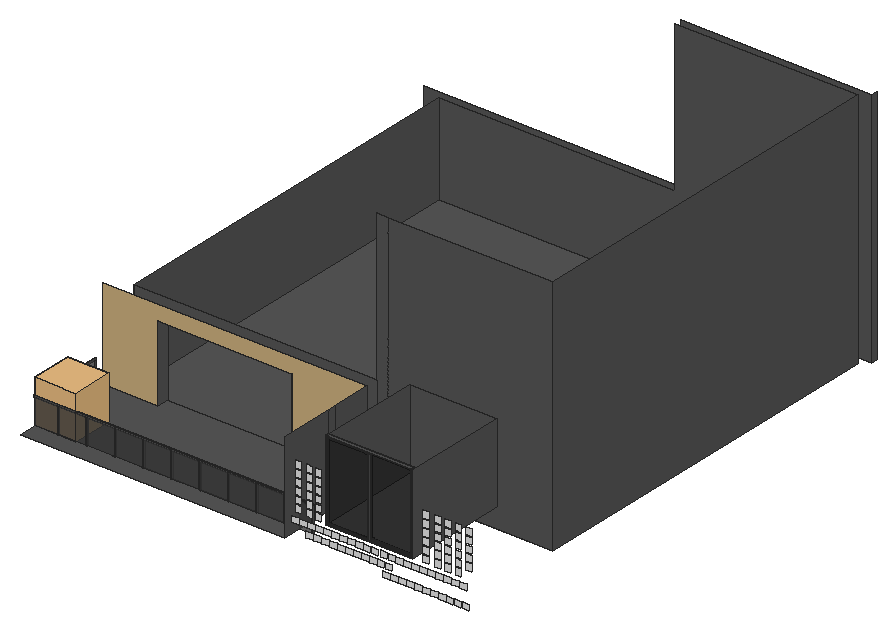
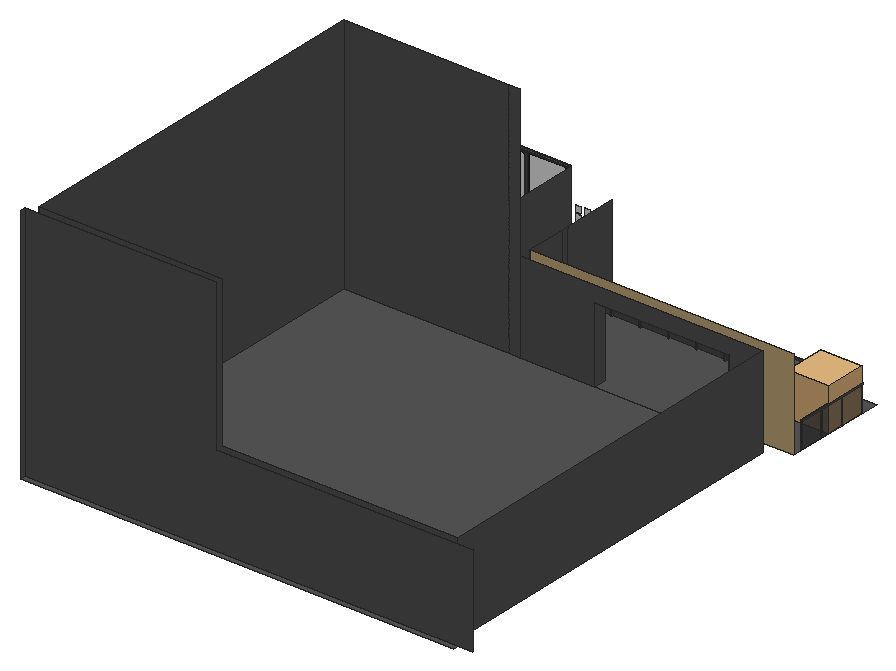
# SketchUp Ruby script. Lengths in inches.
U = 1.inch
M = Sketchup.active_model
def pt(a) = Geom::Point3d.new(a.map { |v| v * U })
def face(e, loops, mat)
  f = e.add_face(loops[0].map { |a| pt(a) })
  loops[1..].each { |l| e.add_face(l.map { |a| pt(a) }).erase! }
  f.material = f.back_material = mat if mat
  f
end
# faces: each face lists its corners as indices into pts; further lists are holes
def faces(e, pts, list, mat = nil) = list.each { |f| face(e, (f[0].is_a?(Array) ? f : [f]).map { |l| l.map { |i| pts[i] } }, mat) }
# xy, xz, yz: faces in a plane at the given z, y or x. An outline is a flat list of corners, or four numbers for a rectangle; further outlines are holes
def ring(l) = l.size == 4 ? [[l[0], l[1]], [l[2], l[1]], [l[2], l[3]], [l[0], l[3]]] : l.each_slice(2).to_a
def flat(e, list, mat, &to3) = list.each { |f| face(e, (f[0].is_a?(Array) ? f : [f]).map { |l| ring(l).map { |u, v| to3.(u, v) } }, mat) }
def xy(e, z, list, mat = nil) = flat(e, list, mat) { |x, y| [x, y, z] }
def xz(e, y, list, mat = nil) = flat(e, list, mat) { |x, z| [x, y, z] }
def yz(e, x, list, mat = nil) = flat(e, list, mat) { |y, z| [x, y, z] }
def lines(e, pts, list) = list.each { |a, b| e.add_line(pt(pts[a]), pt(pts[b])) }
# prism: a flat outline (further loops are holes) pulled along v
def prism(e, loops, v, mat = nil)
  f = face(e, loops, mat); d = Geom::Vector3d.new(v.map { |x| x * U })
  f.pushpull(f.normal.samedirection?(d) ? d.length : -d.length)
end
def box(e, o, s, mat = nil) = prism(e, [[o, [o[0] + s[0], o[1], o[2]], [o[0] + s[0], o[1] + s[1], o[2]], [o[0], o[1] + s[1], o[2]]]], [0, 0, s[2]], mat)
def at(x, y, z, deg = 0) = Geom::Transformation.translation(pt([x, y, z])) * Geom::Transformation.rotation(ORIGIN, Z_AXIS, deg.degrees)
def axes(o, x, y, z) = Geom::Transformation.new([*x, 0, *y, 0, *z, 0, *pt(o).to_a, 1])
def part(name) = M.definitions.add(name)
# library, detail: a bought-in or finely detailed component or shape, given as its bounding box
def library(name, o, s) = part(name).tap { |d| box(d.entities, o, s) }
def detail(e, o, s) = box(e.add_group.entities, o, s)
def put(e, d, t, mat = nil) = e.add_instance(d, t).tap { |i| i.material = mat if mat }
def group(e, t, mat = nil) = e.add_group.tap { |g| g.transformation = t; g.material = mat if mat }.entities
root = M.entities
M.materials.add("Glass_Tinted_Gray").color = [0, 0, 0]
M.materials["Glass_Tinted_Gray"].alpha = 0.125
M.materials.add("[0135_DarkGray]").color = [81, 81, 81]
M.materials.add("[Color M06]").color = [86, 86, 86]
M.materials.add("[Mirror 02]").color = [229, 229, 229]
M.materials.add("[Polished Concrete Old]").color = [229, 229, 229]
M.materials.add("[Terrazzo Light Blue]").color = [196, 214, 227]
M.materials.add("[Translucent Glass Safety]").color = [204, 235, 244]
M.materials["[Translucent Glass Safety]"].alpha = 0.5
M.materials.add("[Translucent_Glass_Gray]").color = [63, 63, 63]
M.materials["[Translucent_Glass_Gray]"].alpha = 0.54
M.materials.add("[Wood Floor Light]").color = [204, 176, 127]
c1 = library("Pot+Plant",[-20.81,-17.08,-0.03],[39.86,39.43,41.33])
c2 = part("Group\#81")
box(c2.entities,[0,0,0],[0.79,39.37,35.43],"[Translucent_Glass_Gray]")
c3 = part("Group\#82")
box(c3.entities,[0,0,0],[0.59,1.57,34.25])
c4 = part("Group\#85")
g1 = group(c4.entities,at(0.55,0.5,0))
put(g1,c2,axes([293.06,0,0],[0,0.84,0],[-0.92977,0,0],[0,0,1]),"[Translucent Glass Safety]")
g2 = group(g1,at(0,33.57,0),"[Translucent Glass Safety]")
box(g2,[0,0,0],[0.73,33.07,35.43],"[Translucent_Glass_Gray]")
put(g1,c2,axes([218.38,0,0],[0,0.84,0],[-0.92977,0,0],[0,0,1]),"[Translucent Glass Safety]")
put(g1,c2,axes([367.73,0,0],[0,0.84,0],[-0.92977,0,0],[0,0,1]),"[Translucent Glass Safety]")
g3 = group(g1,at(31.69,0,0),"[Translucent Glass Safety]")
box(g3,[-30.96,0,0],[30.96,0.66,35.43],"[Translucent_Glass_Gray]")
put(g1,c2,axes([255.72,0,0],[0,0.84,0],[-0.92977,0,0],[0,0,1]),"[Translucent Glass Safety]")
g4 = group(g1,at(181.04,0,0),"[Translucent Glass Safety]")
box(g4,[-36.61,0,0],[36.61,0.66,35.43],"[Translucent_Glass_Gray]")
g5 = group(g1,at(0,0.66,0),"[Translucent Glass Safety]")
box(g5,[0,0,0],[0.73,32.24,35.43],"[Translucent_Glass_Gray]")
g6 = group(g1,at(143.71,0,0),"[Translucent Glass Safety]")
box(g6,[-36.61,0,0],[36.61,0.66,35.43],"[Translucent_Glass_Gray]")
g7 = group(g1,at(69.03,0,0),"[Translucent Glass Safety]")
box(g7,[-36.61,0,0],[36.61,0.66,35.43],"[Translucent_Glass_Gray]")
g8 = group(g1,at(0,67.3,0),"[Translucent Glass Safety]")
box(g8,[0,0,0],[0.73,33.07,35.43],"[Translucent_Glass_Gray]")
put(g1,c3,axes([107.44,0.66,0],[0,1,0],[-0.92977,0,0],[0,0,1]),"[0135_DarkGray]")
put(g1,c3,axes([144.78,0.66,0],[0,1,0],[-0.92977,0,0],[0,0,1]),"[0135_DarkGray]")
put(g1,c3,axes([182.11,0.66,0],[0,1,0],[-0.92977,0,0],[0,0,1]),"[0135_DarkGray]")
put(g1,c3,axes([256.79,0.66,0],[0,1,0],[-0.92977,0,0],[0,0,1]),"[0135_DarkGray]")
put(g1,c3,axes([368.14,0.66,0],[0,1,0],[-0.92977,0,0],[0,0,1]),"[0135_DarkGray]")
put(g1,c3,axes([0.73,98.83,0],[0.92977,0,0],[0,1,0],[0,0,1]),"[0135_DarkGray]")
put(g1,c3,axes([331.46,0.66,0],[0,1,0],[-0.92977,0,0],[0,0,1]),"[0135_DarkGray]")
g9 = group(g1,at(106.37,0,0),"[Translucent Glass Safety]")
box(g9,[-36.61,0,0],[36.61,0.66,35.43],"[Translucent_Glass_Gray]")
put(g1,c2,axes([330.39,0,0],[0,0.84,0],[-0.92977,0,0],[0,0,1]),"[Translucent Glass Safety]")
put(g1,c3,axes([294.125,0.66,0],[0,1,0],[-0.92977,0,0],[0,0,1]),"[0135_DarkGray]")
put(g1,c3,axes([0.73,66.04,0],[0.92977,0,0],[0,1,0],[0,0,1]),"[0135_DarkGray]")
put(g1,c3,axes([0.73,32.31,0],[0.92977,0,0],[0,1,0],[0,0,1]),"[0135_DarkGray]")
put(g1,c3,axes([32.76,0.66,0],[0,1,0],[-0.92977,0,0],[0,0,1]),"[0135_DarkGray]")
put(g1,c3,axes([70.1,0.66,0],[0,1,0],[-0.92977,0,0],[0,0,1]),"[0135_DarkGray]")
put(g1,c3,axes([219.45,0.66,0],[0,1,0],[-0.92977,0,0],[0,0,1]),"[0135_DarkGray]")
g10 = group(c4.entities,at(0,0,34.25))
xy(g10,0,[[0,0,0,100.87,0.55,100.87,0.55,0.5,362.73,0.5,362.73,0],[362.73,0,369.35,0.5],[368.19,0.5,368.6875,1.16],[1.28,1.16,1.28,100.87,1.83,100.87,1.83,1.65,362.73,1.65,362.73,1.16],[362.73,1.16,368.19,1.65]],"[0135_DarkGray]")
xy(g10,1.18,[[368.19,0,368.6875,0.5],[368.6875,0,369.35,0.5],[0.55,0.5,0.55,100.87,1.28,100.87,1.28,1.16,362.73,1.16,362.73,0.5],[368.6875,0.5,369.35,1.16]],"[0135_DarkGray]")
xy(g10,1.97,[[0,0,362.73,0,362.73,1.65,1.83,1.65,1.83,100.87,0,100.87],[362.73,0,368.19,1.65]],"[0135_DarkGray]")
xz(g10,0,[[0,0,362.73,1.97],[362.73,0,369.35,0,369.35,1.18,368.19,1.18,368.19,1.97,362.73,1.97]],"[0135_DarkGray]")
xz(g10,0.5,[[0.55,0,1.28,1.18],[1.28,0,362.73,1.18],[362.73,0,368.19,1.18],[368.19,0,368.6875,1.18],[368.6875,0,369.35,1.18]],"[0135_DarkGray]")
xz(g10,1.16,[[1.28,0,362.73,1.18],[362.73,0,368.19,1.18]],"[0135_DarkGray]")
xz(g10,1.65,[[1.83,0,362.73,1.97],[362.73,0,368.19,1.97]],"[0135_DarkGray]")
xz(g10,100.87,[[0,0,0,1.97,1.83,1.97,1.83,0,1.28,0,1.28,1.18,0.55,1.18,0.55,0]],"[0135_DarkGray]")
yz(g10,0,[[0,0,100.87,1.97]],"[0135_DarkGray]")
yz(g10,0.55,[[0.5,0,100.87,1.18]],"[0135_DarkGray]")
yz(g10,1.28,[[1.16,0,100.87,1.18]],"[0135_DarkGray]")
yz(g10,1.83,[[1.65,0,100.87,1.97]],"[0135_DarkGray]")
yz(g10,362.73,[[0,0,0,1.97,1.65,1.97,1.65,0,1.16,0,1.16,1.18,0.5,1.18,0.5,0]],"[0135_DarkGray]")
yz(g10,368.19,[[1.16,0,1.65,0,1.65,1.97,0,1.97,0,1.18,1.16,1.18],[0.5,0,1.16,1.18]],"[0135_DarkGray]")
yz(g10,368.6875,[[0.5,0,1.16,1.18]],"[0135_DarkGray]")
yz(g10,369.35,[[0,0,0.5,1.18]],"[0135_DarkGray]")
c5 = part("PENTEK_RP Fineline 50S_Sliding_DoorCase_E1")
box(c5.entities,[0,0,0],[1.51,3.66,99.27],"[0135_DarkGray]")
c6 = part("PENTEK_RP Fineline 50S_SlidingDooe_Case_E2")
box(c6.entities,[0,0,0],[96.25,3.66,1.51],"[0135_DarkGray]")
c7 = part("pentek_RP Fineline 50S_SlidingDoor_Case")
put(c7.entities,c5,at(97.76,0,0))
put(c7.entities,c6,at(1.51,0,0))
put(c7.entities,c5,at(0,0,0))
put(c7.entities,c6,at(1.51,0,97.76))
c8 = part("PENTEK_RP Fineline 50S_SlidingDoor_GlazingBead_2")
box(c8.entities,[0,0,0],[0.56,0.59,94.39],"[0135_DarkGray]")
c9 = part("PENTEK_RP Fineline 50S_SlidingDoor_Glass")
box(c9.entities,[0,0,0],[46.58,0.16,94.39],"Glass_Tinted_Gray")
c10 = part("PENTEK_RP Fineline 50S_SlidingDoor_GlazingBead")
box(c10.entities,[0,0,0],[45.47,0.59,0.56],"[0135_DarkGray]")
c11 = part("PENTEK_RP Fineline 50S_SlidingDoor_Leaf_E1")
xy(c11.entities,0,[[0,0,0.93,1.97],[0.93,1.57,1.49,1.97]],"[0135_DarkGray]")
xy(c11.entities,96.25,[[0,0,0.93,0,0.93,1.57,1.49,1.57,1.49,1.97,0,1.97]],"[0135_DarkGray]")
xz(c11.entities,0,[[0,0,0.93,96.25]],"[0135_DarkGray]")
xz(c11.entities,1.57,[[0.93,0,1.49,95.32],[0.93,95.32,1.49,96.25]],"[0135_DarkGray]")
xz(c11.entities,1.97,[[0,0,1.49,96.25]],"[0135_DarkGray]")
yz(c11.entities,0,[[0,0,1.97,96.25]],"[0135_DarkGray]")
yz(c11.entities,0.93,[[0,0,1.57,0.93],[0,0.93,1.57,95.32],[0,95.32,1.57,96.25]],"[0135_DarkGray]")
yz(c11.entities,1.49,[[1.57,0,1.97,95.32],[1.57,95.32,1.97,96.25]],"[0135_DarkGray]")
c12 = part("PENTEK_RP Fineline 50S_SlidingDoor_Leaf_E2")
xy(c12.entities,0,[[0,0,0,1.57,0.56,1.57,0.56,1.97,46.02,1.97,46.02,1.57,46.58,1.57,46.58,0]],"[0135_DarkGray]")
xy(c12.entities,0.93,[[0,0,46.58,1.57]],"[0135_DarkGray]")
xy(c12.entities,1.49,[[0.56,1.57,46.02,1.97]],"[0135_DarkGray]")
xz(c12.entities,0,[[0,0,46.58,0.93]],"[0135_DarkGray]")
xz(c12.entities,1.57,[[0,0,0.56,0.93],[46.02,0,46.58,0.93],[0.56,0.93,46.02,1.49]],"[0135_DarkGray]")
xz(c12.entities,1.97,[[0.56,0,46.02,1.49]],"[0135_DarkGray]")
yz(c12.entities,0,[[0,0,1.57,0.93]],"[0135_DarkGray]")
yz(c12.entities,0.56,[[1.57,0,1.97,0.93],[1.57,0.93,1.97,1.49]],"[0135_DarkGray]")
yz(c12.entities,46.02,[[1.57,0,1.97,0.93],[1.57,0.93,1.97,1.49]],"[0135_DarkGray]")
yz(c12.entities,46.58,[[0,0,1.57,0.93]],"[0135_DarkGray]")
c13 = part("PENTEK_RP Fineline S_SlidingDoor_Leaf1")
put(c13.entities,c8,at(0.93,0,0.93))
put(c13.entities,c8,at(46.96,0,0.93))
put(c13.entities,c9,at(1.49,1.42,0.93))
put(c13.entities,c10,at(1.49,0,0.93))
put(c13.entities,c9,at(1.49,0.59,0.93),"[Terrazzo Light Blue]")
put(c13.entities,c11,at(0,0,0))
put(c13.entities,c11,axes([48.44,0,0],[-1,0,0],[0,1,0],[0,0,1]))
put(c13.entities,c12,axes([0.93,0,96.25],[1,0,0],[0,1,0],[0,0,-1]))
put(c13.entities,c12,at(0.93,0,0))
put(c13.entities,c10,at(1.49,0,94.77))
c14 = part("PENTEK_RP Fineline 50S_SlidingDoor_Leaf2")
put(c14.entities,c9,at(1.49,1.42,0.93))
put(c14.entities,c10,at(1.49,0,94.77))
put(c14.entities,c8,at(46.96,0,0.93))
put(c14.entities,c9,at(1.49,0.59,0.93),"[Mirror 02]")
put(c14.entities,c8,at(0.93,0,0.93))
put(c14.entities,c11,at(0,0,0))
put(c14.entities,c11,axes([48.44,0,0],[-1,0,0],[0,1,0],[0,0,1]))
put(c14.entities,c10,at(1.49,0,0.93))
put(c14.entities,c12,axes([0.93,0,96.25],[1,0,0],[0,1,0],[0,0,-1]))
put(c14.entities,c12,at(0.93,0,0))
c15 = part("PENTEK - Slimmest Steel Sliding Door / Window\#1")
put(c15.entities,c7,at(0,-1.88,-0.09))
put(c15.entities,c13,at(1.51,-2.27,1.42))
put(c15.entities,c14,at(49.32,-0.3,1.42))
xy(root,257.83,[[1.28,10.05,349.9,10.05,349.9,145.99,250.86,145.99,250.86,161.89,74.05,161.89,74.05,145.99,1.28,145.99],[29.53,161.89,582.75,665.33],[19.84,675.01,592.4375,683.05]],"[Color M06]")
xy(root,292.65,[[404.15,10.05,518.59,148.99]],"[Color M06]")
xz(root,10.05,[[479.61,257.42,488.61,264.73],[490.11,257.42,499.11,264.73],[500.61,257.42,509.61,264.73],[511.11,257.42,520.11,264.73],[521.61,257.42,530.61,264.73],
  [532.11,257.42,541.11,264.73],[542.61,257.42,551.61,264.73],[553.11,257.42,562.11,264.73],[563.61,257.42,572.61,264.73],[574.11,257.42,583.11,264.73],
  [584.61,257.42,593.61,264.73],[378.09,268.5,387.09,275.81],[388.59,268.5,397.59,275.81],[399.09,268.5,408.09,275.81],[409.59,268.5,418.59,275.81],
  [420.09,268.5,429.09,275.81],[430.59,268.5,439.59,275.81],[441.09,268.5,450.09,275.81],[451.59,268.5,460.59,275.81],[462.09,268.5,471.09,275.81],
  [472.59,268.5,481.59,275.81],[483.09,268.5,492.09,275.81],[359.62,280.4375,368.62,287.75],[370.12,280.4375,379.12,287.75],[380.62,280.4375,389.62,287.75],
  [391.12,280.4375,400.12,287.75],[401.62,280.4375,410.62,287.75],[412.12,280.4375,421.12,287.75],[422.62,280.4375,431.62,287.75],[433.12,280.4375,442.12,287.75],
  [443.62,280.4375,452.62,287.75],[454.12,280.4375,463.12,287.75],[464.62,280.4375,473.62,287.75],[476.43,280.4375,485.43,287.75],[486.93,280.4375,495.93,287.75],
  [497.43,280.4375,506.43,287.75],[507.93,280.4375,516.93,287.75],[518.43,280.4375,527.43,287.75],[528.93,280.4375,537.93,287.75],[539.43,280.4375,548.43,287.75],
  [549.93,280.4375,558.93,287.75],[560.43,280.4375,569.43,287.75],[570.93,280.4375,579.93,287.75],[581.43,280.4375,590.43,287.75],[364.31,293.74,371.62,302.74],
  [378.93,293.74,386.24,302.74],[390.99,293.74,398.31,302.74],[532.99,293.74,540.31,302.74],[548.43,293.74,555.74,302.74],[561.81,293.74,569.12,302.74],
  [575.62,293.74,582.93,302.74],[364.31,304.24,371.62,313.24],[378.93,304.24,386.24,313.24],[390.99,304.24,398.31,313.24],[532.99,304.24,540.31,313.24],
  [548.43,304.24,555.74,313.24],[561.81,304.24,569.12,313.24],[575.62,304.24,582.93,313.24],[589.18,304.41,596.49,313.41],[364.31,314.74,371.62,323.74],
  [378.93,314.74,386.24,323.74],[390.99,314.74,398.31,323.74],[532.99,314.74,540.31,323.74],[548.43,314.74,555.74,323.74],[561.81,314.74,569.12,323.74],
  [575.62,314.74,582.93,323.74],[589.18,314.91,596.49,323.91],[364.31,325.24,371.62,334.24],[378.93,325.24,386.24,334.24],[390.99,325.24,398.31,334.24],
  [532.99,325.24,540.31,334.24],[548.43,325.24,555.74,334.24],[561.81,325.24,569.12,334.24],[575.62,325.24,582.93,334.24],[589.18,325.41,596.49,334.41],
  [364.31,335.74,371.62,344.74],[378.93,335.74,386.24,344.74],[390.99,335.74,398.31,344.74],[532.99,335.74,540.31,344.74],[548.43,335.74,555.74,344.74],
  [561.81,335.74,569.12,344.74],[575.62,335.74,582.93,344.74],[589.18,335.91,596.49,344.91],[364.31,346.24,371.62,355.24],[378.93,346.24,386.24,355.24],
  [390.99,346.24,398.31,355.24],[532.99,346.24,540.31,355.24],[548.43,346.24,555.74,355.24],[561.81,346.24,569.12,355.24],[575.62,346.24,582.93,355.24],
  [589.18,346.41,596.49,355.41]],"[Polished Concrete Old]")
xz(root,145.99,[[1.28,257.83,74.05,257.83,74.05,357.83,250.86,357.83,250.86,257.83,349.9,257.83,349.9,377.83,1.28,377.83]],"[Wood Floor Light]")
xz(root,148.99,[[404.15,292.65,518.59,397.33]],"[Color M06]")
xz(root,161.89,[[29.53,257.83,29.53,377.83,349.9,377.83,349.9,257.83,250.86,257.83,250.86,357.83,74.05,357.83,74.05,257.83],[349.9,257.83,365.22,575.27],[365.22,257.83,582.75,575.27]],"[Color M06]")
xz(root,665.33,[[29.53,257.83,582.75,257.83,582.75,575.27,340.92,575.27,340.92,377.83,29.53,377.83]],"[Color M06]")
xz(root,675.01,[[1.28,257.83,1.28,377.83,340.92,377.83,340.92,575.27,592.4375,575.27,592.4375,257.83]],"[Color M06]")
yz(root,29.53,[[161.89,257.83,665.33,377.83]],"[Color M06]")
yz(root,74.05,[[145.99,257.83,161.89,357.83]],"[Color M06]")
yz(root,250.86,[[145.99,257.83,161.89,357.83]],"[Color M06]")
yz(root,349.9,[[10.05,257.83,82.9,377.83],[82.9,257.83,92.58,377.83],[92.58,257.83,145.99,377.83]],"[Color M06]")
yz(root,404.15,[[10.05,292.65,148.99,397.33]],"[Color M06]")
yz(root,518.59,[[10.05,292.65,148.99,397.33]],"[Color M06]")
yz(root,582.75,[[161.89,257.83,665.33,575.27]],"[Color M06]")
yz(root,592.4375,[[675.01,257.83,683.05,575.27]],"[Color M06]")
put(root,c1,axes([29.27,57.83,257.88],[1.38,0,0],[0,1.38,0],[0,0,1.38]))
put(root,c4,axes([0,33.1,257.83],[0.99859,0,0],[0,1,0],[0,0,1]),"[Color M06]")
put(root,c15,axes([404.15,12.06,292.74],[1.15276,0,0],[0,1.07,0],[0,0,1.07]),"[Color M06]")
